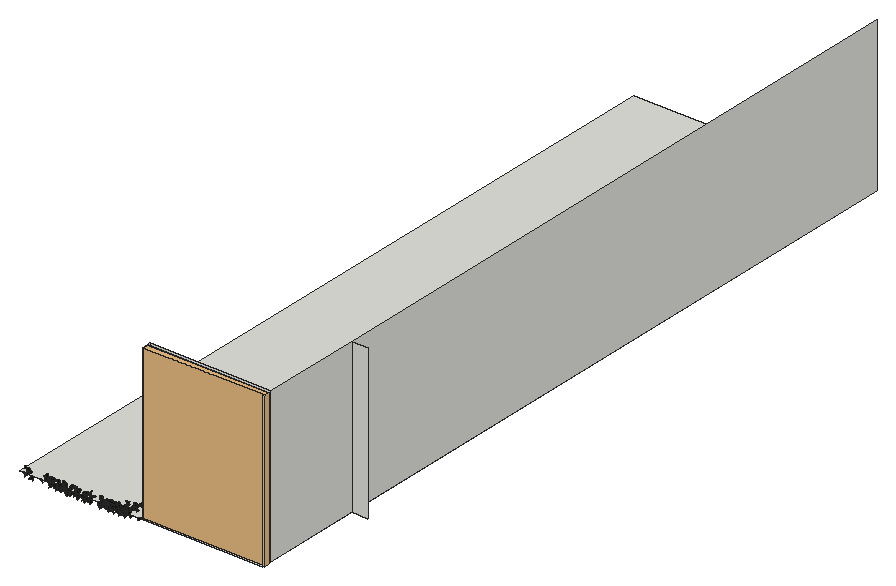
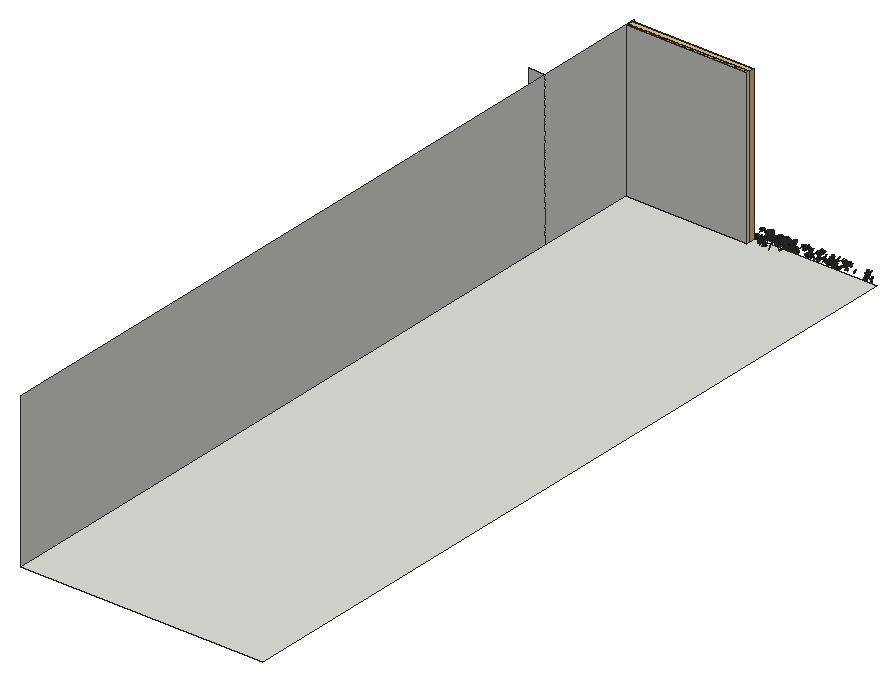
# SketchUp Ruby script. Lengths in inches.
U = 1.inch
M = Sketchup.active_model
def pt(a) = Geom::Point3d.new(a.map { |v| v * U })
def face(e, loops, mat)
  f = e.add_face(loops[0].map { |a| pt(a) })
  loops[1..].each { |l| e.add_face(l.map { |a| pt(a) }).erase! }
  f.material = f.back_material = mat if mat
  f
end
# faces: each face lists its corners as indices into pts; further lists are holes
def faces(e, pts, list, mat = nil) = list.each { |f| face(e, (f[0].is_a?(Array) ? f : [f]).map { |l| l.map { |i| pts[i] } }, mat) }
# xy, xz, yz: faces in a plane at the given z, y or x. An outline is a flat list of corners, or four numbers for a rectangle; further outlines are holes
def ring(l) = l.size == 4 ? [[l[0], l[1]], [l[2], l[1]], [l[2], l[3]], [l[0], l[3]]] : l.each_slice(2).to_a
def flat(e, list, mat, &to3) = list.each { |f| face(e, (f[0].is_a?(Array) ? f : [f]).map { |l| ring(l).map { |u, v| to3.(u, v) } }, mat) }
def xy(e, z, list, mat = nil) = flat(e, list, mat) { |x, y| [x, y, z] }
def xz(e, y, list, mat = nil) = flat(e, list, mat) { |x, z| [x, y, z] }
def yz(e, x, list, mat = nil) = flat(e, list, mat) { |y, z| [x, y, z] }
def lines(e, pts, list) = list.each { |a, b| e.add_line(pt(pts[a]), pt(pts[b])) }
# prism: a flat outline (further loops are holes) pulled along v
def prism(e, loops, v, mat = nil)
  f = face(e, loops, mat); d = Geom::Vector3d.new(v.map { |x| x * U })
  f.pushpull(f.normal.samedirection?(d) ? d.length : -d.length)
end
def box(e, o, s, mat = nil) = prism(e, [[o, [o[0] + s[0], o[1], o[2]], [o[0] + s[0], o[1] + s[1], o[2]], [o[0], o[1] + s[1], o[2]]]], [0, 0, s[2]], mat)
def at(x, y, z, deg = 0) = Geom::Transformation.translation(pt([x, y, z])) * Geom::Transformation.rotation(ORIGIN, Z_AXIS, deg.degrees)
def axes(o, x, y, z) = Geom::Transformation.new([*x, 0, *y, 0, *z, 0, *pt(o).to_a, 1])
def part(name) = M.definitions.add(name)
# library, detail: a bought-in or finely detailed component or shape, given as its bounding box
def library(name, o, s) = part(name).tap { |d| box(d.entities, o, s) }
def detail(e, o, s) = box(e.add_group.entities, o, s)
def put(e, d, t, mat = nil) = e.add_instance(d, t).tap { |i| i.material = mat if mat }
def group(e, t, mat = nil) = e.add_group.tap { |g| g.transformation = t; g.material = mat if mat }.entities
root = M.entities
M.materials.add("efeu1").color = [18, 25, 13]
M.materials.add("efeu2").color = [43, 57, 29]
c1 = part("ivyleaf_9")
p = [[1.54,2.16,1.25],[1.36,2.04,1.19],[-0.21,0.99,0.68],[-0.71,1.11,0.82],[-0.85,0.86,0.67],[-0.8,0.17,0.21],
  [-0.9,-0.01,0.1],[-0.67,-0.16,-0.02],[-0.08,-0.08,-0.05],[-0.03,-0.6,-0.4],[0.65,-0.88,-0.66],[0.83,-0.6,-0.49],
  [1.29,-0.42,-0.43],[1.8125,-0.07,-0.26],[1.21,0.44,0.15]]
faces(c1.entities,p,[[0,1,2,3,4,5,6,7,8,9,10,11,12,13,14]],"efeu1")
c2 = part("ivyleaf_10")
p = [[0,0.5,-0.03],[-0.0625,2.02,-0.43],[-0.19,2.01,-0.46],[-0.54,1.05,-0.29],[-0.52,0.625,-0.18],[-0.83,0.76,-0.28],
  [-1.16,0.64,-0.33],[-1.15,0.33,-0.24],[-0.77,-0.39,0.02],[-0.3,-0.51,0.16],[0.04,-0.48,0.23],[-0.02,2.01,-0.4375],
  [-0.06,2.01,-0.43],[0.04,-0.49,0.23],[0.67,-0.49,0.14],[1.38,0.36,-0.2],[1.375,0.51,-0.24],[0.81,0.65,-0.19],
  [0.62,0.59,-0.15],[0.6,1.09,-0.28],[0.5,1.23,-0.31]]
faces(c2.entities,p,[[0,1,2,3,4,5,6,7,8,9,10],[11,12,0,13,14,15,16,17,18,19,20]],"efeu2")
c3 = library("Wall Panel 104-26",[-34.24,-2.8,0],[68.48,2.8,108.01])
xy(root,253.9375,[[0,223.4375,133.125,223.4375,133.125,227.3125,66.5625,227.3125,66.5625,229.125,133.125,229.125,133.125,643.9375,0,643.9375]])
xz(root,227.3125,[[66.5625,253.9375,133.125,337.75]])
xz(root,229.125,[[66.5625,253.9375,133.125,337.75]])
xz(root,284.3125,[[133.125,253.9375,142.16,337.75]])
yz(root,66.5625,[[227.3125,253.9375,229.125,337.75]])
yz(root,133.125,[[223.4375,253.9375,227.3125,337.75],[229.125,253.9375,284.3125,337.75],[284.3125,253.9375,643.9375,337.75]])
put(root,c1,axes([54.88,220.89,257.22],[-0.36156,-0.34519,-0.01075],[0.00935,0.00577,-0.49988],[0.34523,-0.36168,0.00229]))
put(root,c1,axes([50.71,221.04,255.21],[-0.24436,-0.36569,0.23783],[-0.00467,-0.27039,-0.42056],[0.43619,-0.20776,0.12873]))
put(root,c1,axes([49.23,220.99,256.99],[-0.27233,-0.40293,0.11611],[0.01006,-0.14469,-0.4785],[0.41921,-0.25828,0.08692]))
put(root,c1,axes([40.06,220.81,258.32],[-0.05555,-0.47858,-0.13371],[0.06287,0.12669,-0.47958],[0.49291,-0.07009,0.0461]))
put(root,c1,axes([19.33,220.83,255.86],[-0.01123,-0.49254,-0.08532],[0.01833,0.08488,-0.4924],[0.49954,-0.01418,0.01615]))
put(root,c1,axes([39.34,220.6,254.58],[0.45035,-0.21022,-0.05472],[-0.04636,0.03003,-0.49694],[0.21222,0.45266,0.00756]))
put(root,c1,axes([38.79,220.83,258.12],[-0.49761,-0.04878,-0.00249],[0.00278,-0.00286,-0.49998],[0.04876,-0.49761,0.00312]))
put(root,c1,axes([58.56,220.95,255.58],[-0.46669,-0.08903,0.15581],[-0.11964,-0.16922,-0.45503],[0.13375,-0.462,0.13664]))
put(root,c1,axes([54.51,220.92,256.3125],[-0.40504,-0.12713,0.26416],[-0.25533,-0.0684,-0.42441],[0.14405,-0.47871,-0.00951]))
put(root,c1,axes([37.67,220.92,255.14],[0.18062,-0.3162,0.34263],[0.19258,-0.28404,-0.36364],[0.42461,0.26333,0.01918]))
put(root,c1,axes([50.76,220.63,254.62],[0.04525,0.42174,-0.26473],[-0.10346,-0.25206,-0.41924],[-0.48708,0.09272,0.06445]))
put(root,c1,axes([38.91,221.01,255.36],[0.01562,-0.46334,0.18727],[0.04144,-0.18551,-0.46246],[0.49803,0.02997,0.0326]))
put(root,c1,axes([31.54,220.92,255.4],[-0.01909,-0.49958,-0.0072],[0.0004,0.00719,-0.49995],[0.49964,-0.01909,0.00013]))
put(root,c1,axes([35.89,220.86,255.9],[0.08263,-0.48969,-0.05811],[-0.00061,0.05882,-0.49653],[0.49313,0.08212,0.00912]))
put(root,c1,axes([58.46,220.97,256.01],[-0.48381,-0.11569,-0.05045],[0.08018,-0.12739,-0.47681],[0.09747,-0.46945,0.14182]))
put(root,c1,axes([59.29,220.47,258.75],[0.3425,0.35935,-0.0597],[-0.04057,-0.04381,-0.49642],[-0.36201,0.34489,-0.00085]))
put(root,c1,axes([45.7,220.57,254.34],[0.39113,0.1552,-0.27006],[-0.25369,-0.09279,-0.42075],[-0.18072,0.46616,0.00616]))
put(root,c1,axes([37.4,220.6,254.87],[-0.44313,-0.09329,0.21198],[0.21144,0.02381,0.45247],[-0.09451,0.49064,0.01835]))
put(root,c1,axes([24.99,221.08,255.27],[-0.33932,-0.32644,0.16821],[-0.08144,-0.15643,-0.46786],[0.35809,-0.34491,0.05299]))
put(root,c1,axes([33.81,220.82,257.02],[-0.0366,-0.45457,-0.205],[0.01552,0.20441,-0.45604],[0.49842,-0.03975,-0.00086]))
put(root,c1,axes([30.42,220.47,254.98],[0.43511,0.22701,0.09563],[0.08544,0.04296,-0.49077],[-0.23104,0.44342,-0.0014]))
put(root,c1,axes([38.01,221.05,254.68],[-0.33747,-0.36081,0.07701],[-0.02095,-0.08545,-0.4922],[0.36834,-0.33543,0.04255]))
put(root,c1,axes([33.09,221.14,256.27],[-0.25874,-0.33868,0.26144],[-0.03273,-0.28896,-0.40673],[0.42659,-0.22759,0.12736]))
put(root,c1,axes([59.33,221.01,258.25],[-0.28152,-0.41299,-0.01358],[0.01661,0.0051,-0.4997],[0.41288,-0.2818,0.01085]))
put(root,c1,axes([47.7,221.02,255.61],[0.09386,-0.46544,0.15671],[0.03549,-0.1527,-0.47479],[0.48983,0.10025,0.00437]))
put(root,c1,axes([26.01,221,258.71],[-0.46342,-0.15066,0.11202],[-0.10521,-0.0387,-0.48727],[0.15549,-0.47519,0.00417]))
put(root,c1,axes([22.7,221.01,258.43],[0.0354,-0.49806,0.02622],[-0.00021,-0.0263,-0.49931],[0.49875,0.03534,-0.00207]))
put(root,c1,axes([51.58,221,257.93],[-0.18076,-0.46195,-0.06264],[0.01339,0.06201,-0.49596],[0.46599,-0.18098,-0.01004]))
put(root,c1,axes([37.22,221.02,257.69],[-0.15617,-0.4717,-0.05572],[0.01183,0.05477,-0.49685],[0.47484,-0.15651,-0.00595]))
put(root,c1,axes([49.24,220.9375,258.08],[-0.42533,0.16737,-0.20268],[0.15976,-0.14154,-0.45215],[-0.20873,-0.44939,0.06692]))
put(root,c1,axes([56.51,221.06,254.61],[0.1124,-0.35086,0.33803],[0.22056,-0.27268,-0.35637],[0.43442,0.22922,0.09347]))
put(root,c1,axes([19.39,221.06,258.4],[-0.06496,-0.49492,0.02887],[0.00201,-0.02938,-0.49913],[0.49576,-0.06473,0.00581]))
put(root,c1,axes([49.5625,220.71,257.21],[0.48261,-0.09055,0.09429],[0.09042,-0.02926,-0.49088],[0.09441,0.49086,-0.01187]))
put(root,c1,axes([52.76,220.4,256.22],[0.27542,0.23088,0.34762],[0.1782,0.31155,-0.34811],[-0.37735,0.31564,0.08933]))
put(root,c1,axes([23.92,220.95,256.58],[-0.26065,0.11916,0.40971],[-0.42646,-0.08866,-0.24551],[0.01415,-0.47743,0.14785]))
put(root,c1,axes([48.15,220.66,255.41],[0.36021,-0.17281,-0.30064],[-0.24799,0.17463,-0.3975],[0.24238,0.43548,0.0401]))
put(root,c1,axes([46.7,220.72,258.41],[-0.32386,0.3175,0.2105],[-0.19034,0.10445,-0.4504],[-0.32998,-0.37186,0.05321]))
put(root,c1,axes([52.41,220.93,254.21],[0.32056,-0.38131,0.04296],[0.0294,-0.03141,-0.49815],[0.3826,0.32189,0.00228]))
put(root,c1,axes([59.02,220.69,258.74],[-0.2653,0.42203,0.03884],[-0.01944,0.03365,-0.49849],[-0.42336,-0.26601,-0.00144]))
put(root,c1,axes([49.625,220.97,254.46],[0.19925,-0.45821,-0.01852],[-0.0059,0.01762,-0.49965],[0.45855,0.19933,0.00162]))
put(root,c1,axes([55.59,220.84,255.76],[0.37356,-0.32364,-0.07557],[-0.05532,0.05156,-0.49425],[0.32771,0.37762,0.00271]))
put(root,c1,axes([18.72,221.07,258.1],[0.15218,-0.47463,0.03967],[0.00773,-0.03918,-0.4984],[0.47622,0.1523,-0.00459]))
put(root,c1,axes([40.42,220.74,256.68],[0.16826,-0.30985,-0.35451],[-0.02367,0.37043,-0.335],[0.47024,0.12952,0.10998]))
put(root,c1,axes([61.38,221.19,257.85],[-0.28117,-0.41052,0.0491],[0.02551,-0.07649,-0.49345],[0.41266,-0.27499,0.06396]))
put(root,c1,axes([24.85,221.19,255.01],[-0.24711,-0.43051,0.05997],[-0.03609,-0.04842,-0.49634],[0.43317,-0.24963,-0.00715]))
put(root,c1,axes([26.32,220.95,255.74],[0.13603,-0.45173,-0.16563],[-0.01341,0.1685,-0.47056],[0.48095,0.13247,0.03373]))
put(root,c1,axes([60.86,221.31,258.32],[0.1381,-0.2208,-0.42682],[0.22176,-0.3647,0.26041],[-0.42632,-0.26123,-0.0028]))
put(root,c1,axes([16.64,221.26,257.33],[-0.27293,-0.37293,0.19088],[-0.11332,-0.1536,-0.46213],[0.40332,-0.29552,-0.00067]))
put(root,c1,axes([31.91,220.71,259.04],[0.46781,-0.00719,-0.17637],[-0.17239,0.08882,-0.46086],[0.03795,0.492,0.08062]))
put(root,c1,axes([18.85,221.08,258.22],[0.05389,-0.48973,-0.08523],[-0.00045,0.08568,-0.4926],[0.49709,0.05316,0.0088]))
put(root,c1,axes([19.35,221.11,257.77],[-0.19312,-0.44498,-0.12125],[0.03635,0.11635,-0.48491],[0.45976,-0.19611,-0.01259]))
put(root,c1,axes([47.09,220.59,256.83],[-0.01141,0.45126,0.21502],[-0.03257,0.21394,-0.45074],[-0.49881,-0.02429,0.02451]))
put(root,c1,axes([47.71,220.94,254.78],[0.38814,-0.31315,-0.03587],[-0.02675,0.02397,-0.49871],[0.31406,0.38906,0.00185]))
put(root,c1,axes([53.97,220.93,258.65],[-0.33527,0.36986,-0.0282],[-0.09011,-0.11809,-0.47743],[-0.35983,-0.31505,0.14584]))
put(root,c1,axes([32.47,221.27,258.35],[-0.04318,-0.47971,0.13421],[-0.01197,-0.13367,-0.48165],[0.49799,-0.04481,0.00006]))
put(root,c1,axes([40.28,220.9,258.04],[0.33049,-0.34002,-0.15864],[-0.04256,0.17606,-0.46604],[0.37278,0.32154,0.08743]))
put(root,c1,axes([58.04,221.2,257.01],[-0.20284,-0.45505,-0.04221],[0.02945,0.03307,-0.49803],[0.45606,-0.20453,0.01339]))
put(root,c1,axes([45.98,221.06,258.46],[0.22171,-0.44511,-0.05212],[-0.01764,0.04943,-0.49724],[0.44781,0.22233,0.00622]))
put(root,c1,axes([53.8125,221.1875,256.125],[-0.48239,-0.12435,0.0429],[-0.03027,-0.05374,-0.49618],[0.12802,-0.4813,0.04432]))
put(root,c1,axes([53.32,221.1875,255.51],[-0.45807,-0.19617,0.04109],[-0.03811,-0.0154,-0.49831],[0.19677,-0.45965,-0.00085]))
put(root,c1,axes([49.24,220.9,257.29],[0.47064,-0.14126,0.09242],[0.08779,-0.029,-0.49138],[0.14419,0.47875,-0.0025]))
put(root,c1,axes([18.55,221.3,254.42],[-0.35515,-0.33546,0.10647],[-0.03628,-0.11556,-0.48511],[0.35007,-0.3523,0.05775]))
put(root,c1,axes([20.18,221.02,258.64],[0.26168,-0.41698,-0.08745],[-0.00312,0.10075,-0.48973],[0.42604,0.25686,0.05013]))
put(root,c1,axes([61.15,220.71,258.28],[0.21695,0.44981,-0.02462],[-0.05337,-0.00147,-0.49714],[-0.44731,0.21834,0.04738]))
put(root,c1,axes([40.42,221.25,254.48],[-0.10852,-0.48723,0.02887],[0.00011,-0.0296,-0.49912],[0.48808,-0.10833,0.00653]))
put(root,c1,axes([18.625,221.17,257.52],[-0.49535,-0.06789,0.00425],[-0.00185,-0.01779,-0.49968],[0.068,-0.49505,0.01737]))
put(root,c1,axes([28.16,221.2,255.81],[0.00441,-0.49983,-0.01225],[0.00245,0.01227,-0.49984],[0.49997,0.00434,0.00255]))
put(root,c1,axes([33.4,220.93,255.52],[0.10202,-0.35871,-0.33305],[0.08173,0.34791,-0.34968],[0.48261,0.01691,0.12963]))
put(root,c1,axes([56.79,221.17,255.53],[0.17131,-0.46906,0.02522],[0.0086,-0.02371,-0.49936],[0.46966,0.17153,-0.00005]))
put(root,c1,axes([38.21,220.85,257.2],[0.14039,0.44366,-0.18293],[-0.07978,-0.16637,-0.46471],[-0.47321,0.15966,0.02408]))
put(root,c1,axes([48.875,221.02,257.26],[0.2728,-0.40484,-0.10811],[0.00668,0.13318,-0.48189],[0.41897,0.26147,0.07807]))
put(root,c1,axes([46.53,221.2,258.19],[-0.055,-0.49337,-0.0597],[0.00475,0.05954,-0.49642],[0.49694,-0.05517,-0.00186]))
put(root,c1,axes([58.88,221.17,258.26],[0.10813,-0.48754,-0.02473],[0.0032,0.02604,-0.49931],[0.48816,0.10782,0.00875]))
put(root,c2,axes([45.54,220.99,253.9],[-0.02055,0.49545,-0.06407],[0.0007,-0.06409,-0.49587],[-0.49958,-0.02047,0.00194]))
put(root,c1,axes([41.01,220.63,256.32],[0.13008,0.10086,0.47213],[0.29289,0.37222,-0.16022],[-0.38379,0.31824,0.03776]))
put(root,c1,axes([47.66,221.22,255.57],[-0.46634,-0.17794,-0.02942],[0.0276,0.0102,-0.49913],[0.17823,-0.46715,0.00031]))
put(root,c1,axes([60.25,220.91,258.72],[-0.23084,0.44335,-0.01229],[-0.07086,-0.05054,-0.49237],[-0.43783,-0.22557,0.08616]))
put(root,c1,axes([58.73,220.92,257.6875],[-0.22963,0.44367,-0.02055],[-0.05716,-0.05247,-0.49394],[-0.44046,-0.2245,0.07482]))
put(root,c1,axes([18.69,221.43,254.57],[-0.20497,-0.33341,0.31117],[-0.012,-0.33709,-0.36909],[0.4559,-0.15877,0.13018]))
put(root,c1,axes([37.13,221.22,254.32],[0.04515,-0.49762,-0.01843],[-0.00733,0.01784,-0.49963],[0.4979,0.04538,-0.00569]))
put(root,c1,axes([25.46,221.36,255.39],[-0.31693,-0.34809,0.1685],[-0.10943,-0.12823,-0.47072],[0.37092,-0.33525,0.0051]))
put(root,c1,axes([24.68,221.3,255.11],[-0.16238,-0.47224,0.02489],[-0.00699,-0.02391,-0.49938],[0.47285,-0.16253,0.00116]))
put(root,c1,axes([6.36,221.16,258.42],[-0.36761,-0.12621,-0.24925],[0.24635,0.07402,-0.37745],[0.15776,-0.40966,0.00859]))
put(root,c1,axes([54.59,221.23,257.86],[-0.47778,-0.14631,-0.01778],[0.01886,-0.00086,-0.49964],[0.14618,-0.47811,0.00634]))
put(root,c1,axes([33.93,221.32,254.37],[-0.28764,-0.40811,0.02662],[-0.0066,-0.02791,-0.49918],[0.40892,-0.28752,0.01067]))
put(root,c1,axes([33.17,221.35,254.53],[-0.02929,-0.47681,0.14764],[0.0219,-0.14898,-0.47679],[0.49866,-0.02146,0.02961]))
put(root,c1,axes([30.45,221.1875,258.8],[0.08476,-0.48841,-0.06536],[-0.00144,0.06608,-0.49561],[0.49276,0.0842,0.00979]))
put(root,c1,axes([26.74,221.41,257.93],[-0.27762,-0.38115,0.16627],[0.00879,-0.20526,-0.45584],[0.41575,-0.25018,0.12067]))
put(root,c1,axes([39.68,221.03,254.64],[0.25229,-0.39469,-0.17484],[-0.02744,0.18744,-0.46273],[0.43081,0.24308,0.07291]))
put(root,c1,axes([53.3,221.23,256.18],[0.05323,-0.49605,-0.03321],[0.00613,0.03405,-0.4988],[0.49712,0.05269,0.00971]))
put(root,c1,axes([15.24,221.34,257.59],[0.14785,-0.35811,0.31607],[0.12012,-0.29235,-0.38743],[0.46229,0.19049,-0.00042]))
put(root,c1,axes([29.72,221.27,254.75],[-0.36512,-0.31412,-0.13423],[0.13065,0.05313,-0.4797],[0.31563,-0.38536,0.04328]))
put(root,c1,axes([51.15,221.18,257.4],[0.21155,-0.45301,-0.00497],[0.03862,0.0235,-0.49795],[0.45139,0.2103,0.04493]))
put(root,c1,axes([49.3,221.14,255.48],[0.08729,-0.46839,-0.15164],[0.01032,0.15571,-0.47502],[0.49221,0.0798,0.03685]))
put(root,c1,axes([46.3,220.92,258.9],[0.26802,0.31503,-0.28093],[-0.21939,-0.18033,-0.41152],[-0.3606,0.34386,0.04156]))
put(root,c1,axes([25.92,221.42,255.42],[-0.06141,-0.42672,0.25326],[0.04652,-0.25902,-0.42514],[0.49403,-0.02866,0.07151]))
put(root,c1,axes([18.625,221.14,257.01],[-0.29095,-0.21277,-0.34652],[0.27824,0.20656,-0.36044],[0.29654,-0.40257,-0.00179]))
put(root,c1,axes([60.3,221.37,256.14],[-0.13523,-0.47535,0.07587],[0.03403,-0.08805,-0.49101],[0.48016,-0.12764,0.05617]))
put(root,c1,axes([62.67,220.87,255.1],[0.23414,0.4229,-0.12779],[-0.06591,-0.10957,-0.48337],[-0.43685,0.2432,0.00444]))
put(root,c1,axes([19.21,221.2,256.47],[0.14727,-0.47595,-0.04226],[0.02738,0.05256,-0.49648],[0.47703,0.14392,0.04155]))
put(root,c2,axes([45.62,221.1,254.54],[0.24239,-0.43375,-0.05575],[-0.02351,0.05072,-0.49686],[0.43669,0.24349,0.0042]))
put(root,c1,axes([51.71,221,257.78],[-0.05686,0.45369,-0.20231],[-0.01325,-0.20494,-0.45588],[-0.49658,-0.04648,0.03533]))
put(root,c1,axes([25.05,221.23,256.46],[-0.49833,0.0389,-0.01236],[0.00925,-0.0398,-0.49833],[-0.03975,-0.49689,0.03895]))
put(root,c1,axes([52.62,221.06,255.24],[-0.42477,0.2392,0.11115],[-0.09271,0.06187,-0.48742],[-0.24694,-0.43469,-0.00821]))
put(root,c1,axes([48.79,221.14,256.01],[0.30487,-0.39304,-0.05075],[-0.02067,0.04818,-0.49724],[0.39576,0.30529,0.01313]))
put(root,c1,axes([59.8125,221.07,256.35],[0.18935,-0.4038,-0.22604],[-0.10973,0.19808,-0.44578],[0.44956,0.21843,-0.0136]))
put(root,c1,axes([24.57,221.24,255.34],[0.17443,-0.46813,0.02079],[0.0987,0.01502,-0.48993],[0.45807,0.17502,0.09765]))
put(root,c1,axes([55.17,221.09,257.84],[0.40326,-0.29517,-0.01592],[-0.00907,0.01455,-0.49971],[0.29546,0.40332,0.00639]))
put(root,c1,axes([50.5,221.33,254.74],[-0.36973,-0.33457,-0.03692],[0.02546,0.0269,-0.49863],[0.33564,-0.37059,-0.00285]))
put(root,c1,axes([60.05,221.33,255.9375],[-0.38003,-0.05658,-0.31997],[0.32406,-0.10201,-0.36685],[-0.02377,-0.4862,0.11421]))
put(root,c1,axes([25.875,221.3,257.23],[-0.05791,-0.49239,-0.06478],[0.02919,0.06173,-0.49532],[0.49578,-0.06115,0.0216]))
put(root,c1,axes([21.38,221.39,254.33],[-0.05685,-0.49197,0.06876],[0.00551,-0.06983,-0.49507],[0.49673,-0.05554,0.01336]))
put(root,c1,axes([57.22,221.34,255.94],[-0.13355,-0.48046,-0.03642],[0.01191,0.0345,-0.49867],[0.48169,-0.13406,0.00223]))
put(root,c1,axes([50.04,220.98,257.75],[-0.27167,0.41094,0.08558],[-0.10948,0.02905,-0.487],[-0.40523,-0.28335,0.07419]))
put(root,c1,axes([50.67,220.78,258.52],[0.27363,0.41079,0.07984],[0.0069,0.09096,-0.49161],[-0.41842,0.27014,0.04411]))
put(root,c1,axes([50.41,221.25,257.07],[-0.44349,0.14374,0.18071],[-0.21112,-0.09391,-0.44341],[-0.09353,-0.46959,0.14399]))
put(root,c1,axes([20.67,221.43,255.48],[-0.15605,-0.46643,0.08994],[0.00793,-0.09722,-0.49039],[0.47496,-0.15163,0.03774]))
put(root,c1,axes([29.56,221.43,257.28],[-0.04262,-0.48196,0.12607],[0.01655,-0.12783,-0.4831],[0.49791,-0.03701,0.02685]))
put(root,c1,axes([52.71,220.87,255.36],[0.42933,0.25398,0.03421],[0.02812,0.01966,-0.49882],[-0.25472,0.43024,0.00259]))
put(root,c1,axes([25.53,221.27,257.19],[0.26419,-0.41557,0.08661],[0.06309,-0.06244,-0.49206],[0.41979,0.27093,0.01945]))
put(root,c1,axes([24.77,220.77,256.11],[0.3149,0.19965,0.33313],[0.25349,0.21927,-0.37103],[-0.29425,0.40257,0.03688]))
put(root,c1,axes([28.23,221.39,254.27],[-0.34651,-0.36023,-0.01286],[0.01373,0.00464,-0.49979],[0.3602,-0.34672,0.00667]))
put(root,c1,axes([63.55,220.94,258.47],[-0.13554,0.48086,0.02005],[0.00058,0.02099,-0.49956],[-0.48128,-0.1354,-0.00625]))
put(root,c1,axes([26.59,221.3,256.67],[-0.01078,-0.48832,-0.10689],[0.01882,0.10644,-0.48818],[0.49953,-0.01454,0.01608]))
put(root,c1,axes([59.21,221.22,257.72],[-0.44968,0.19778,-0.09312],[0.08199,-0.04483,-0.49119],[-0.20264,-0.45703,0.00789]))
put(root,c1,axes([25.15,221.39,256.12],[-0.10932,-0.48781,-0.00951],[0.0052,0.00859,-0.4999],[0.48788,-0.1094,0.00319]))
put(root,c1,axes([60.14,221.39,257.55],[-0.11617,-0.48569,-0.02462],[-0.00616,0.02678,-0.49924],[0.48628,-0.11569,-0.0122]))
put(root,c1,axes([45.78,221.17,254.53],[0.19426,-0.41981,-0.18981],[-0.06849,0.17739,-0.46243],[0.4556,0.20566,0.01141]))
put(root,c1,axes([59.34,221.38,257.87],[-0.39216,-0.27486,-0.14375],[0.14975,0.03515,-0.47575],[0.27163,-0.4162,0.05475]))
put(root,c1,axes([24.29,221.27,256.12],[-0.4811,0.08719,0.10458],[-0.10642,-0.00122,-0.48854],[-0.08493,-0.49234,0.01973]))
put(root,c1,axes([6.1,221.33,258.09],[-0.27403,-0.23429,-0.27507],[0.2916,0.08149,-0.34444],[0.24616,-0.35734,0.1018]))
put(root,c1,axes([56.1875,221.47,254.95],[-0.27841,-0.41484,0.01996],[0.03248,-0.04571,-0.49685],[0.41405,-0.27536,0.0524]))
put(root,c1,axes([34.23,221.46,257.64],[-0.00702,-0.49105,0.09394],[0.01568,-0.09411,-0.49081],[0.4997,-0.00394,0.01672]))
put(root,c1,axes([25.37,221.43,255.28],[-0.45731,-0.20084,0.02297],[-0.01199,-0.02977,-0.49897],[0.20179,-0.45692,0.02241]))
put(root,c1,axes([45.7,220.96,254.23],[-0.13214,0.47563,0.07945],[-0.01253,0.07897,-0.49357],[-0.48206,-0.13243,-0.00895]))
put(root,c1,axes([45.04,221.53,255.09],[-0.05314,-0.46995,0.16223],[-0.01619,-0.16143,-0.47294],[0.4969,-0.05552,0.00194]))
put(root,c1,axes([58.43,221.41,254.06],[0.13812,-0.47679,0.05997],[0.01753,-0.05736,-0.49639],[0.48022,0.13922,0.00087]))
put(root,c1,axes([46.74,221.33,254.6875],[-0.09776,0.31925,-0.37219],[0.07114,-0.36626,-0.33285],[-0.48516,-0.11803,0.02619]))
put(root,c1,axes([13.24,221.41,255.32],[0.21717,-0.43583,0.11354],[0.03959,-0.10709,-0.48679],[0.44863,0.22042,-0.012]))
put(root,c1,axes([58.88,221.5,254.6],[-0.03733,-0.48451,-0.11771],[-0.0085,-0.1174,0.48595],[-0.49853,0.03828,0.00053]))
put(root,c1,axes([48.79,221.34,255.48],[0.21745,-0.44901,-0.03321],[-0.01902,0.02769,-0.49887],[0.44984,0.21823,-0.00504]))
put(root,c1,axes([16.45,221.38,257.71],[-0.49879,-0.00169,0.03477],[-0.03476,-0.00257,-0.49878],[0.00186,-0.49999,0.00245]))
put(root,c1,axes([59.29,221.35,257.62],[0.27175,-0.41965,-0.00684],[-0.00581,0.00439,-0.49995],[0.41967,0.2718,-0.00249]))
put(root,c1,axes([32.45,221.34,257.33],[0.21484,-0.44511,-0.07564],[-0.01596,0.07623,-0.4939],[0.45121,0.21463,0.01854]))
put(root,c1,axes([60.67,221.27,255.16],[0.00731,0.37786,-0.32737],[-0.05356,-0.32493,-0.37623],[-0.49707,0.04057,0.03572]))
put(root,c1,axes([18.79,221.04,258.03],[-0.15684,0.46862,0.07614],[-0.02716,0.0712,-0.49416],[-0.47399,-0.15914,0.00312]))
put(root,c1,axes([51.39,220.9,258.375],[0.3303,0.3623,0.09821],[-0.01977,0.14742,-0.47736],[-0.37485,0.31146,0.11171]))
put(root,c1,axes([25.29,221.1,256.91],[0.49958,0.00453,0.02006],[0.01998,0.00811,-0.49953],[-0.00485,0.49991,0.00792]))
put(root,c1,axes([58.52,220.92,257.38],[-0.02626,0.42136,0.26789],[-0.0933,0.25939,-0.41715],[-0.49052,-0.0719,0.065]))
put(root,c1,axes([45.5,220.91,255.46],[0.34303,0.33707,0.13681],[0.05678,0.13612,-0.47775],[-0.35932,0.3433,0.05511]))
put(root,c1,axes([16.4,221.08,258.88],[0.15655,-0.26636,-0.39312],[-0.08693,0.39087,-0.29944],[0.46684,0.1621,0.07607]))
put(root,c1,axes([40.42,221.18,258.76],[-0.26179,0.42424,-0.03852],[-0.00972,-0.05115,-0.49728],[-0.42588,-0.25962,0.03503]))
put(root,c1,axes([36.13,221.43,254.46],[-0.44251,0.08195,-0.21788],[0.20348,-0.09115,-0.44754],[-0.11307,-0.48474,0.04732]))
put(root,c1,axes([60.86,221.125,257.9],[-0.14553,0.47698,-0.03624],[0.00402,-0.03666,-0.49864],[-0.47834,-0.14542,0.00684]))
put(root,c1,axes([49.97,221.125,258.4],[0.49858,0.01525,-0.03441],[-0.0346,0.00592,-0.49877],[-0.0148,0.49973,0.00696]))
put(root,c1,axes([56.27,221.49,254.47],[-0.35968,-0.32022,-0.1345],[0.11198,0.07637,-0.48128],[0.32877,-0.37633,0.01678]))
put(root,c1,axes([42.03,221.04,257.75],[0.49869,0.03568,-0.00572],[-0.01559,0.14107,-0.47943],[-0.0326,0.47836,0.14181]))
put(root,c1,axes([61.35,221.14,258.08],[0.43774,0.11418,-0.21294],[-0.20445,-0.05981,-0.45235],[-0.12877,0.4831,-0.00568]))
put(root,c1,axes([56.19,221.02,256.81],[-0.00426,-0.06982,0.49508],[0.01815,0.49475,0.06993],[-0.49965,0.01857,-0.00168]))
put(root,c1,axes([58.75,221.12,255.29],[0.02129,0.49677,-0.05261],[-0.05835,-0.04983,-0.49408],[-0.49613,0.02717,0.05585]))
put(root,c1,axes([61.09,221.52,257.5],[-0.40894,-0.09935,-0.26999],[0.2768,-0.00797,-0.41632],[0.07842,-0.48996,0.06152]))
put(root,c1,axes([32.34,221.43,256.85],[0.12446,-0.46965,-0.11805],[0.00351,0.12276,-0.48468],[0.48425,0.11982,0.03386]))
put(root,c1,axes([50.34,221.19,257.02],[0.45745,-0.16183,-0.12064],[-0.08034,0.12817,-0.47657],[0.18517,0.4554,0.09126]))
put(root,c1,axes([27.32,221.7,254.14],[-0.29776,-0.37421,0.14597],[-0.00347,-0.1793,-0.46673],[0.40166,-0.27896,0.10418]))
put(root,c1,axes([16.2,221.32,257.36],[0.1177,-0.39525,-0.28271],[0.0581,0.30025,-0.39557],[0.48246,0.06026,0.11661]))
put(root,c1,axes([44.51,221.3125,254.02],[0.40612,-0.1065,0.27151],[0.25951,-0.08049,-0.41974],[0.13311,0.48185,-0.0101]))
put(root,c1,axes([3.89,221.32,255.58],[0.44222,-0.1229,0.08362],[0.08249,-0.02523,-0.4446],[0.13548,0.41652,-0.00226]))
put(root,c1,axes([49.57,221.3,255.88],[-0.18156,0.44544,-0.13647],[0.06839,-0.11939,-0.48069],[-0.46082,-0.19322,-0.01758]))
put(root,c1,axes([7.1,221.17,254.24],[-0.11036,0.48576,0.04309],[-0.01053,0.0418,-0.49814],[-0.48756,-0.11086,0.001]))
put(root,c1,axes([54.46,221.8,255.65],[-0.45608,-0.15111,0.13841],[0.10676,-0.46348,-0.15423],[0.17491,-0.11113,0.45504]))
put(root,c1,axes([51.57,221.6,254.55],[-0.07863,-0.05614,-0.49058],[-0.29713,-0.39137,0.09241],[-0.39437,0.30607,0.02818]))
put(root,c1,axes([51.98,221.32,257.93],[-0.1618,0.11411,0.45913],[-0.37722,0.26174,-0.19799],[-0.28553,-0.41045,0.00139]))
put(root,c1,axes([18.15,221.25,255.77],[-0.28261,0.35384,0.21196],[-0.137,0.16183,-0.45282],[-0.38905,-0.31402,0.00549]))
put(root,c1,axes([24.95,221.49,255.06],[0.24374,-0.42312,-0.10751],[-0.02327,0.11036,-0.48711],[0.43595,0.24246,0.0341]))
put(root,c1,axes([57.04,221.5625,255.36],[0.25333,-0.43089,0.01265],[0.01315,-0.00694,-0.49978],[0.43087,0.25355,0.00781]))
put(root,c1,axes([55.01,221.12,254.68],[0.05873,0.47755,0.13601],[0.0179,0.13483,-0.48114],[-0.49622,0.06138,-0.00126]))
put(root,c1,axes([61.05,221.34,257.98],[0.26508,0.32752,-0.26919],[-0.16743,-0.21079,-0.42135],[-0.38949,0.31352,-0.00208]))
put(root,c1,axes([33.39,221.67,254.21],[-0.32638,-0.32815,-0.18921],[0.19441,0.06923,-0.45542],[0.32509,-0.37085,0.0824]))
put(root,c1,axes([51.26,221.53,253.98],[-0.46135,0.18564,-0.05194],[0.04449,-0.02854,-0.4972],[-0.18756,-0.46338,0.00981]))
put(root,c1,axes([6.21,221.4,256.02],[-0.05343,0.39471,-0.18305],[-0.01245,-0.1783,-0.41248],[-0.46659,-0.04044,0.03197]))
put(root,c1,axes([50.45,221.51,254.7],[-0.41288,0.27518,-0.06171],[0.00985,-0.09528,-0.49074],[-0.28184,-0.40645,0.07325]))
put(root,c1,axes([60.56,221.38,256.99],[-0.2666,0.41916,-0.05687],[0.01888,-0.05537,-0.49657],[-0.42258,-0.26691,0.0137]))
put(root,c1,axes([55.82,221.48,254.82],[-0.42721,0.24001,0.09944],[-0.10874,0.0086,-0.48796],[-0.23594,-0.43855,0.04485]))
put(root,c1,axes([61.57,221.18,256.18],[0.15064,0.47507,0.04019],[0.00625,0.04017,-0.49834],[-0.47673,0.15065,0.00617]))
put(root,c1,axes([57.02,221.43,255.41],[-0.3853,0.31785,0.02271],[-0.01875,0.01297,-0.49948],[-0.31811,-0.38575,0.00193]))
put(root,c1,axes([58.61,221.19,257.03],[0.39175,0.30975,0.02423],[-0.00408,0.04412,-0.49803],[-0.31067,0.39001,0.0371]))
put(root,c1,axes([57.04,221.63,255.04],[-0.26322,-0.03544,-0.42363],[0.42414,0.01176,-0.26452],[0.02871,-0.4986,0.02387]))
put(root,c1,axes([61.66,221.4,258.3],[0.21981,0.3386,-0.29502],[-0.1752,-0.23778,-0.40344],[-0.41351,0.28073,0.01411]))
put(root,c1,axes([54.55,221.22,257.12],[-0.15879,0.43711,0.18363],[-0.05229,0.17633,-0.46495],[-0.47122,-0.16686,-0.01028]))
put(root,c1,axes([48.42,221.26,254.16],[0.44584,0.2243,-0.03029],[-0.02572,-0.01628,-0.49907],[-0.22487,0.44657,-0.00298]))
put(root,c1,axes([60.59,221.3,257.17],[0.17903,0.45055,-0.12228],[-0.04631,-0.11318,-0.48481],[-0.46455,0.18492,0.00121]))
put(root,c1,axes([4.24,221.57,258.49],[0.28346,-0.34631,-0.02109],[-0.00012,0.02534,-0.45163],[0.37465,0.26202,0.01581]))
put(root,c1,axes([56.71,221.53,254.24],[-0.3549,0.34763,-0.05659],[-0.04696,-0.12632,-0.4815],[-0.34906,-0.33645,0.12231]))
put(root,c1,axes([32.71,221.79,254.11],[0.0028,-0.4956,0.06611],[-0.01435,-0.06616,-0.4954],[0.49979,0.00088,-0.01459]))
put(root,c1,axes([23.01,221.66,254],[-0.03948,-0.00485,0.49842],[-0.49722,0.03538,-0.03904],[-0.03489,-0.49872,-0.00762]))
put(root,c1,axes([57.74,221.38,256.36],[0.00955,-0.00031,0.49991],[0.49858,0.03641,-0.0095],[-0.0364,0.49867,0.001]))
put(root,c1,axes([25.74,221.21,257.77],[0.07576,0.45343,0.19662],[-0.01696,0.20119,-0.45742],[-0.49394,0.06264,0.04587]))
put(root,c1,axes([51.81,221.3125,255.91],[0.40436,0.29311,0.02413],[0.01692,0.01777,-0.4994],[-0.29362,0.40468,0.00445]))
put(root,c1,axes([51.45,221.59,253.67],[0.18809,-0.31252,0.34199],[-0.11719,0.325,0.36145],[-0.44821,-0.21612,0.04901]))
put(root,c1,axes([58.36,221.29,256.06],[0.29083,0.39825,0.08254],[0.05642,0.06099,-0.49305],[-0.40278,0.2961,-0.00946]))
put(root,c1,axes([24.82,221.33,255.71],[0.08274,-0.07625,-0.48718],[-0.35759,0.33086,-0.11252],[0.33953,0.36704,0.00021]))
put(root,c1,axes([39.08,221.4,254.09],[0.30232,0.3866,-0.09564],[-0.06727,-0.06878,-0.49066],[-0.39253,0.30953,0.01043]))
put(root,c1,axes([5.91,221.32,256.56],[0.31035,0.3152,0.08886],[-0.01857,0.12825,-0.43192],[-0.35221,0.27097,0.10107]))
put(root,c1,axes([25.03,221.55,254.42],[0.45732,-0.18463,-0.08229],[-0.07631,0.0308,-0.49318],[0.18718,0.46364,-0.00001]))
put(root,c1,axes([48.63,221.83,255.08],[-0.01769,-0.49216,-0.08643],[0.27194,0.06307,-0.41481],[0.41921,-0.06168,0.26544]))
put(root,c1,axes([25.26,221.32,256.75],[0.17927,0.45994,0.07947],[0.0044,0.08346,-0.49297],[-0.46674,0.17744,0.02587]))
put(root,c1,axes([59.3125,221.52,255.35],[-0.11125,0.48573,-0.04114],[-0.05259,-0.05392,-0.49429],[-0.48462,-0.10565,0.06309]))
put(root,c1,axes([53.68,221.34,255.25],[0.04616,0.4207,0.26623],[-0.01646,0.26851,-0.42146],[-0.49759,0.03014,0.03864]))
put(root,c1,axes([46.73,221.51,257.01],[-0.01891,-0.12998,-0.48244],[0.09009,0.47399,-0.13123],[0.49145,-0.09189,0.00549]))
put(root,c1,axes([4.2,221.67,254.3],[-0.17059,0.38753,-0.12348],[0.06426,-0.10387,-0.43493],[-0.43299,-0.1681,-0.0159]))
put(root,c1,axes([24.17,221.55,254.16],[0.13684,0.46828,-0.10949],[-0.01428,-0.10983,-0.48758],[-0.4807,0.13657,-0.01669]))
put(root,c1,axes([51.38,221.56,253.98],[-0.04792,0.49748,-0.01468],[0.00351,-0.01441,-0.49978],[-0.49769,-0.048,-0.00211]))
put(root,c1,axes([6.46,221.68,256.15],[-0.15203,0.09927,0.41542],[-0.35443,0.22772,-0.17914],[-0.26829,-0.35709,0.00125]))
put(root,c1,axes([50.7,221.8,257.79],[0.21181,-0.43371,-0.13051],[0.22339,0.22537,-0.3864],[0.394,0.10538,0.28924]))
put(root,c1,axes([7.7,221.9,254.31],[0.14779,-0.46765,-0.09726],[-0.01073,0.09853,-0.49008],[0.47754,0.14694,0.01909]))
put(root,c2,axes([24.33,221.79,254.32],[-0.23743,-0.43675,-0.05365],[0.05683,0.03001,-0.49585],[0.43635,-0.24156,0.03539]))
put(root,c1,axes([59.59,221.75,255.48],[0.49698,0.02506,-0.04885],[-0.04869,-0.00424,-0.49761],[-0.02535,0.49935,-0.00178]))
put(root,c1,axes([6.64,221.66,256.84],[0.32124,0.31332,0.05285],[0.039,0.03579,-0.4493],[-0.34058,0.29963,-0.0016]))
put(root,c1,axes([54.52,222.26,254.2],[-0.12365,-0.4844,-0.00841],[0.3456,-0.08211,-0.35188],[0.33952,-0.09283,0.35512]))
put(root,c1,axes([66.06,221.78,254.4],[0.16696,-0.02258,0.47076],[0.43785,0.19221,-0.14607],[-0.17437,0.46103,0.08396]))
put(root,c1,axes([55.78,222.45,256.9],[-0.23543,-0.42253,0.12664],[-0.0707,-0.10555,-0.48359],[0.4354,-0.24561,-0.01004]))
put(root,c1,axes([47.59,222.1875,254.05],[0.35995,-0.31584,-0.1438],[0.29529,0.38759,-0.11215],[0.18232,-0.00419,0.46556]))
put(root,c1,axes([49.79,222.06,257.22],[0.43562,-0.19541,-0.14849],[0.10696,0.42343,-0.24345],[0.22089,0.18035,0.41071]))
put(root,c1,axes([63.6,222.23,258.83],[0.46815,0.15321,0.08579],[0.0817,0.02619,-0.49258],[-0.15543,0.47523,-0.00052]))
put(root,c1,axes([54.49,223.26,257.36],[-0.48554,-0.11937,-0.00218],[0.0019,0.00138,-0.49999],[0.11938,-0.48554,-0.00088]))
put(root,c1,axes([54.37,223.3,255.71],[0.05321,-0.49599,0.03403],[0.00808,-0.03336,-0.49882],[0.49709,0.05364,0.00447]))
put(root,c1,axes([54.32,223.62,254.72],[-0.43916,0.2302,-0.06435],[0.00891,-0.11875,-0.48561],[-0.23886,-0.42767,0.1002]))
put(root,c1,axes([56.9,225.34,258.21],[0.28967,-0.34843,0.21139],[0.12645,-0.1697,-0.453],[0.38743,0.31591,-0.01019]))
put(root,c1,axes([57.55,225.24,258.11],[0.06619,-0.33016,-0.36961],[0.00125,0.373,-0.33297],[0.4956,0.04316,0.05021]))
put(root,c1,axes([50.71,226,255.06],[-0.12415,-0.44451,-0.19236],[0.15538,0.15153,-0.45044],[0.45874,-0.17162,0.10052]))
put(root,c3,axes([99.875,227.3125,253.5],[0.97199,0,0],[0,1,0],[0,0,0.78]))
put(root,c1,axes([59.93,226.43,257.15],[-0.38589,0.25463,-0.1904],[0.13086,-0.14569,-0.46005],[-0.28977,-0.40489,0.0458]))
put(root,c1,axes([58.51,226.2,254.88],[0.38984,0.08306,0.30187],[0.28919,0.08921,-0.39801],[-0.11998,0.48491,0.02152]))
put(root,c1,axes([61.23,226.52,255.8125],[0.45502,-0.20345,0.03955],[0.03557,-0.01734,-0.49843],[0.20418,0.45641,-0.00131]))
put(root,c1,axes([60.52,226.5625,255.57],[0.33724,-0.34465,-0.13222],[-0.08541,0.10137,-0.48211],[0.35913,0.34776,0.0095]))
put(root,c1,axes([60.11,226.625,256.44],[0.41523,-0.25152,0.11968],[0.11236,-0.04533,-0.4851],[0.25487,0.42975,0.01888]))
put(root,c1,axes([55.96,226.4,254.92],[0.20758,-0.03767,-0.45331],[-0.39625,0.22972,-0.20054],[0.22338,0.4425,0.06552]))
put(root,c1,axes([60.48,226.54,258.23],[0.49076,0.07623,0.05782],[0.05878,-0.00174,-0.49653],[-0.0755,0.49415,-0.01067]))
put(root,c1,axes([59.14,226.74,255.34],[0.49116,0.03956,-0.08481],[-0.08804,0.04169,-0.49042],[-0.03173,0.49669,0.04792]))
put(root,c1,axes([60.41,226.74,257.16],[0.08862,0.48315,0.09335],[0.03105,0.08917,-0.491],[-0.4911,0.09282,-0.0142]))
put(root,c1,axes([63.27,227.1,258.7],[-0.09365,0.42232,-0.25076],[-0.00628,-0.25628,-0.42928],[-0.49111,-0.07726,0.05331]))
put(root,c1,axes([62.26,227.11,257.52],[0.47477,-0.02814,0.15429],[0.15536,0.01716,-0.47494],[0.02143,0.49891,0.02503]))
put(root,c1,axes([61.34,227.94,256.5],[-0.4374,0.237,0.05013],[-0.05543,0.0028,-0.49691],[-0.23581,-0.44026,0.02383]))
put(root,c1,axes([60.75,227.8,255.94],[-0.1118,0.45343,0.1786],[-0.13783,0.14634,-0.45781],[-0.46744,-0.1516,0.09228]))
